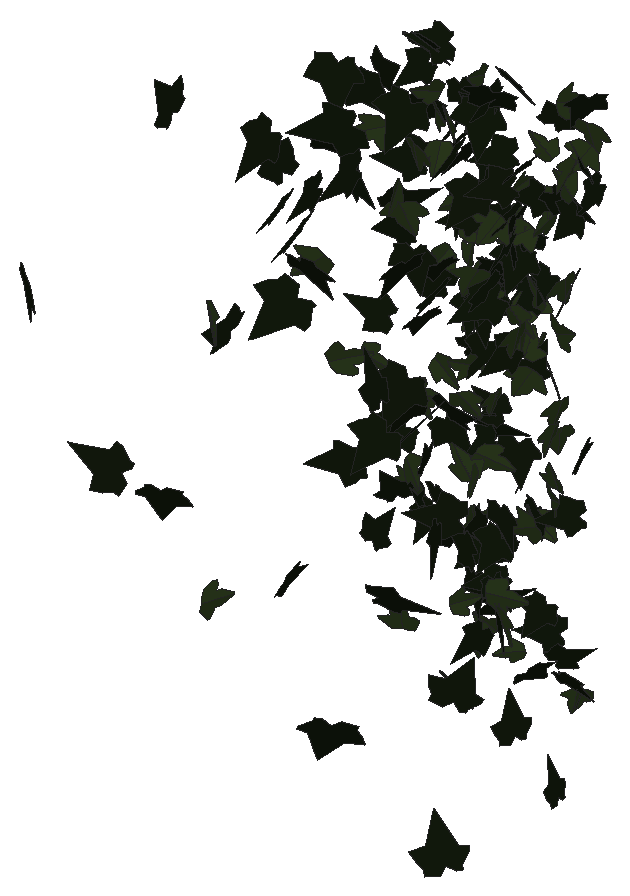
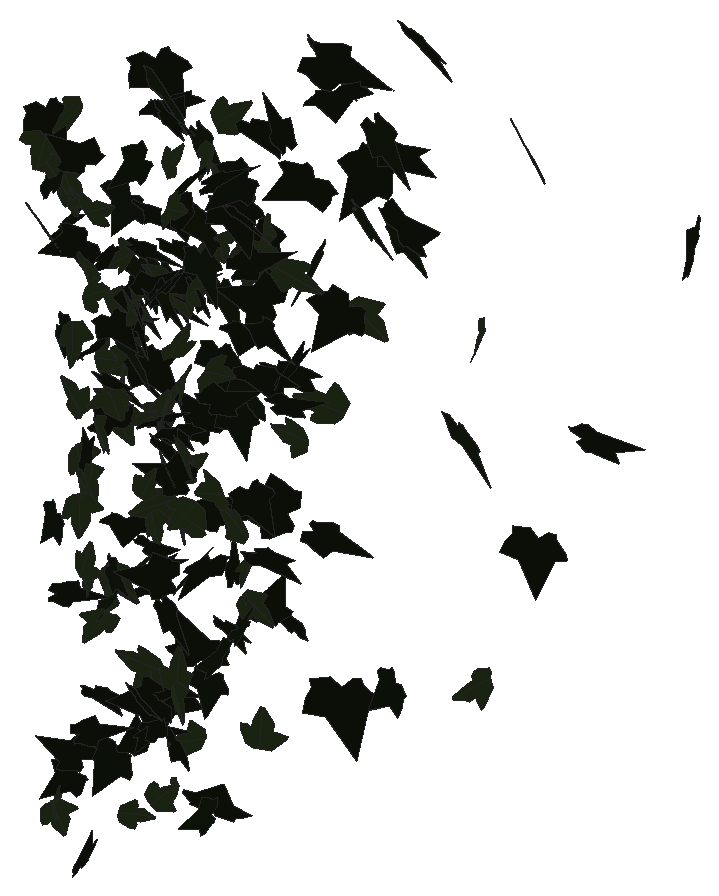
# SketchUp Ruby script. Lengths in millimetres.
U = 1.mm
M = Sketchup.active_model
def pt(a) = Geom::Point3d.new(a.map { |v| v * U })
def face(e, loops, mat)
  f = e.add_face(loops[0].map { |a| pt(a) })
  loops[1..].each { |l| e.add_face(l.map { |a| pt(a) }).erase! }
  f.material = f.back_material = mat if mat
  f
end
# faces: each face lists its corners as indices into pts; further lists are holes
def faces(e, pts, list, mat = nil) = list.each { |f| face(e, (f[0].is_a?(Array) ? f : [f]).map { |l| l.map { |i| pts[i] } }, mat) }
# xy, xz, yz: faces in a plane at the given z, y or x. An outline is a flat list of corners, or four numbers for a rectangle; further outlines are holes
def ring(l) = l.size == 4 ? [[l[0], l[1]], [l[2], l[1]], [l[2], l[3]], [l[0], l[3]]] : l.each_slice(2).to_a
def flat(e, list, mat, &to3) = list.each { |f| face(e, (f[0].is_a?(Array) ? f : [f]).map { |l| ring(l).map { |u, v| to3.(u, v) } }, mat) }
def xy(e, z, list, mat = nil) = flat(e, list, mat) { |x, y| [x, y, z] }
def xz(e, y, list, mat = nil) = flat(e, list, mat) { |x, z| [x, y, z] }
def yz(e, x, list, mat = nil) = flat(e, list, mat) { |y, z| [x, y, z] }
def lines(e, pts, list) = list.each { |a, b| e.add_line(pt(pts[a]), pt(pts[b])) }
# prism: a flat outline (further loops are holes) pulled along v
def prism(e, loops, v, mat = nil)
  f = face(e, loops, mat); d = Geom::Vector3d.new(v.map { |x| x * U })
  f.pushpull(f.normal.samedirection?(d) ? d.length : -d.length)
end
def box(e, o, s, mat = nil) = prism(e, [[o, [o[0] + s[0], o[1], o[2]], [o[0] + s[0], o[1] + s[1], o[2]], [o[0], o[1] + s[1], o[2]]]], [0, 0, s[2]], mat)
def at(x, y, z, deg = 0) = Geom::Transformation.translation(pt([x, y, z])) * Geom::Transformation.rotation(ORIGIN, Z_AXIS, deg.degrees)
def axes(o, x, y, z) = Geom::Transformation.new([*x, 0, *y, 0, *z, 0, *pt(o).to_a, 1])
def part(name) = M.definitions.add(name)
# library, detail: a bought-in or finely detailed component or shape, given as its bounding box
def library(name, o, s) = part(name).tap { |d| box(d.entities, o, s) }
def detail(e, o, s) = box(e.add_group.entities, o, s)
def put(e, d, t, mat = nil) = e.add_instance(d, t).tap { |i| i.material = mat if mat }
def group(e, t, mat = nil) = e.add_group.tap { |g| g.transformation = t; g.material = mat if mat }.entities
root = M.entities
M.materials.add("efeu1").color = [18, 25, 13]
M.materials.add("efeu2").color = [43, 57, 29]
c1 = part("ivyleaf_9")
p = [[39.1,54.8,31.7],[34.5,51.8,30.2],[-5.3,25.2,17.3],[-17.9,28.3,20.9],[-21.6,21.7,17],[-20.2,4.3,5.3],
  [-22.9,-0.3,2.5],[-17.1,-4,-0.6],[-2,-2.1,-1.2],[-0.7,-15.4,-10.1],[16.6,-22.3,-16.7],[21.1,-15.1,-12.5],
  [32.7,-10.7,-11],[46.1,-1.8,-6.6],[30.8,11.2,3.8]]
faces(c1.entities,p,[[0,1,2,3,4,5,6,7,8,9,10,11,12,13,14]],"efeu1")
c2 = part("ivyleaf_10")
p = [[0,12.8,-0.8],[-1.5,51.3,-10.9],[-4.9,51,-11.6],[-13.6,26.5,-7.3],[-13.2,15.9,-4.6],[-21.1,19.3,-7.2],
  [-29.5,16.3,-8.3],[-29.2,8.3,-6.2],[-19.7,-9.8,0.5],[-7.6,-13,4],[1,-12.2,5.8],[-0.4,51.1,-11.1],
  [-1.5,51.1,-10.9],[1,-12.4,5.9],[16.9,-12.4,3.5],[35.1,9.1,-5.1],[35,12.9,-6.1],[20.5,16.4,-4.9],
  [15.8,15,-3.8],[15.3,27.6,-7.1],[12.8,31.3,-7.8]]
faces(c2.entities,p,[[0,1,2,3,4,5,6,7,8,9,10],[11,12,0,13,14,15,16,17,18,19,20]],"efeu2")
put(root,c1,axes([55.6,82.1,1285.6],[0.45869,-0.23293,-1.38227],[1.53626,-0.57264,0.43901],[-0.75134,-1.31306,0.05375]))
put(root,c1,axes([225.6,151.3,899.1],[-1.14115,-0.48465,-0.89648],[-0.97651,-0.4038,1.05345],[-0.76956,1.23107,-0.00739]))
put(root,c1,axes([576.3,245.3,1354.5],[-1.46005,-0.85692,0.36484],[-0.37109,-0.20185,-1.47187],[1.07395,-1.23475,-0.01259]))
put(root,c1,axes([463.1,305.7,1644.5],[-1.71291,0.10789,-0.47473],[0.57263,-0.0846,-1.40741],[-0.15763,-1.47969,0.04586]))
put(root,c1,axes([205.4,303.4,780.9],[1.00786,0.77267,-0.61847],[-0.55474,-0.41924,-1.13113],[-1.07246,0.94298,0.00388]))
put(root,c1,axes([527.4,323.5,1454.6],[-1.0107,1.1156,-0.43445],[0.31599,-0.3488,-1.38956],[-1.426,-0.86799,0.00001]))
put(root,c1,axes([528.1,326.9,1379.9],[1.66772,0.20054,-0.333],[-0.40215,-0.04725,-1.38161],[-0.25136,1.40616,0.00107]))
put(root,c1,axes([582.2,346.2,385.4],[0.82118,1.01451,-0.90267],[-0.64285,-0.73341,-1.21719],[-1.5269,0.85439,0.027]))
put(root,c2,axes([275.1,366.2,1172.6],[-0.51795,1.04749,-0.55022],[0.2633,-0.5062,-1.13022],[-1.41929,-0.47618,-0.00888]))
put(root,c1,axes([620,369,1593.3],[-1.46779,0.67443,-0.22377],[0.23179,-0.11868,-1.37921],[-0.83535,-1.21797,0.01049]))
put(root,c1,axes([686.9,367.3,692.6],[1.08384,-0.27376,1.03511],[1.27629,-0.06449,-0.91492],[0.27817,1.36255,0.16467]))
put(root,c1,axes([174.5,373.7,1565.1],[-0.42554,0.80332,1.20672],[-0.55224,1.11874,-0.8756],[-1.68015,-0.57118,-0.01783]))
put(root,c2,axes([257,379.8,530.6],[-0.05912,-0.19143,-1.2224],[0.57322,1.12885,-0.19541],[1.39643,-0.47149,0.02846]))
put(root,c1,axes([646.6,428.1,1007.3],[-1.48699,-0.57457,-0.02828],[0.02999,0.01418,-1.34748],[0.70119,-1.21909,-0.00234]))
put(root,c1,axes([547.2,445.3,1630.5],[-0.34453,-0.17863,-1.47318],[-1.08704,-1.17881,0.31374],[-1.44778,0.92759,0.11501]))
put(root,c1,axes([792.8,429.2,128.3],[-1.64579,-0.13251,0.15894],[0.19426,0.00487,1.35546],[-0.16125,1.35833,0.01065]))
put(root,c1,axes([366.3,469.9,1386.5],[-0.90124,0.86965,-0.39727],[0.28644,-0.32165,-1.14071],[-1.13071,-0.77464,0.02766]))
put(root,c1,axes([585.6,487.8,1039.8],[-0.40845,-0.99324,0.75452],[0.28417,0.7177,1.04812],[-1.49496,0.40779,-0.00691]))
put(root,c1,axes([229.2,480.3,1060.4],[-0.89362,1.14725,0.43552],[-0.30714,0.35593,-1.361],[-1.46527,-0.77428,0.01967]))
put(root,c1,axes([766.5,488.1,445.8],[-1.05162,-0.07692,0.96033],[1.16947,-0.19731,0.8446],[0.11751,1.27527,0.18861]))
put(root,c1,axes([412.2,514.1,1416.8],[-1.25714,0.56506,-0.40164],[0.406,-0.22803,-1.17459],[-0.74195,-1.08219,0.03779]))
put(root,c1,axes([652.6,489.2,978.4],[-0.30811,1.18465,-0.34746],[-0.08994,0.33955,1.21127],[1.50347,0.26308,0.00126]))
put(root,c1,axes([694.8,524.5,773.9],[-0.81085,0.21669,-1.02259],[1.20492,-0.26673,-0.69844],[-0.4177,-1.19008,-0.02966]))
put(root,c1,axes([610.8,539.4,1061],[-1.48604,-0.67855,-0.32666],[0.34772,0.1596,-1.39432],[0.85043,-1.25097,-0.0007]))
put(root,c1,axes([347.3,505,549.5],[-0.36462,0.48619,-0.98361],[-0.67259,0.81487,0.57029],[1.15735,0.62673,0.02154]))
put(root,c1,axes([613.8,529.9,1317.5],[-0.37333,1.14013,-0.69859],[0.18967,-0.68145,-1.18026],[-1.62024,-0.34248,0.0228]))
put(root,c2,axes([397.8,538.7,1250],[-0.85455,-0.45354,0.88487],[-0.8633,-0.53302,-0.83335],[0.85222,-0.99474,0.0431]))
put(root,c1,axes([318.7,524.2,1423.2],[-0.09591,0.19519,1.39451],[-1.21961,0.97588,-0.19295],[-1.20982,-0.99925,0.08396]))
put(root,c2,axes([446.1,537.5,1047.3],[-0.38963,-0.3588,1.10004],[0.87719,0.83256,0.4803],[-1.106,0.78672,-0.00659]))
put(root,c1,axes([420.8,568,1666.1],[-0.57355,-1.23514,-0.35463],[0.11207,0.34435,-1.32111],[1.56374,-0.4777,-0.03539]))
put(root,c1,axes([458.1,567,822.9],[-0.24261,-0.25527,-1.12314],[-0.9252,-0.82881,0.32265],[-1.05759,0.78362,-0.02461]))
put(root,c1,axes([699.1,577.4,775.7],[-0.74553,-0.13299,1.02767],[-1.23175,-0.19223,-0.62524],[0.28466,-1.18008,-0.01397]))
put(root,c1,axes([484,599,649],[-0.6613,0.57536,0.71293],[0.6009,-0.51545,0.79047],[0.94242,0.73239,-0.00375]))
put(root,c1,axes([638.6,591.8,1232.9],[-0.60337,1.21146,0.07928],[-0.03851,0.07275,-1.30852],[-1.48064,-0.49556,0.00172]))
put(root,c1,axes([648.7,616,974],[0.15352,-0.46219,1.0981],[1.07593,-0.70629,-0.39834],[0.97728,0.85019,0.26604]))
put(root,c2,axes([452.4,621.3,1027],[-0.13538,0.05172,-1.06693],[1.19144,-0.42966,-0.1224],[-0.52796,-0.98287,-0.00263]))
put(root,c1,axes([541.4,634.5,1591.7],[-1.45326,-0.64338,-0.29041],[0.3319,0.10722,-1.35341],[0.79465,-1.22139,0.03416]))
put(root,c2,axes([512,637.7,1400.4],[-0.16625,0.60985,-0.88681],[-0.0257,-0.89523,-0.6124],[-1.3128,-0.0597,0.12429]))
put(root,c1,axes([690.4,633.3,673.7],[0.02582,-1.10176,0.25788],[0.00471,0.25799,1.10193],[-1.38047,-0.01973,0.00858]))
put(root,c1,axes([658.6,626.8,1531.2],[-0.90319,0.84807,-0.33833],[0.27204,-0.25445,-1.12574],[-1.08021,-0.77317,-0.00062]))
put(root,c1,axes([799.1,630.4,321.5],[-0.63448,-0.81045,0.65983],[0.63538,0.43799,0.94846],[-1.1054,0.71694,0.16645]))
put(root,c2,axes([523.6,639,1360.8],[-1.3266,-0.54908,-0.30435],[0.34779,0.11046,-1.2178],[0.68238,-1.12375,0.029]))
put(root,c2,axes([510.8,649.8,450.9],[-1.22373,-0.38729,-0.06213],[-0.07073,-0.02233,1.07523],[-0.47328,1.00473,-0.00005]))
put(root,c1,axes([730.3,634.6,1254.8],[-0.74057,1.1525,0.22615],[-0.19479,0.17124,-1.30117],[-1.41956,-0.62474,0.06056]))
put(root,c1,axes([397.4,637.8,1395.4],[1.01337,-0.60092,-0.79642],[-0.75489,0.50265,-1.0246],[0.95482,1.03517,0.0352]))
put(root,c1,axes([467.3,656.4,1100.5],[-0.79559,-0.58876,-0.57812],[-0.51954,-0.391,0.87857],[-0.86225,0.77884,0.00405]))
put(root,c2,axes([684.7,652.4,829.5],[0.7233,-0.92555,-0.33551],[-0.18829,0.29943,-1.09874],[1.18622,0.61188,0.03017]))
put(root,c1,axes([721.6,667.1,1222.8],[-1.54651,-0.15024,0.27481],[-0.32026,-0.11522,-1.27389],[0.2084,-1.29195,0.08166]))
put(root,c1,axes([678.8,678,480.3],[-0.04303,-0.00885,-1.11829],[0.50108,-1.04076,-0.00472],[-1.26901,-0.41066,0.03605]))
put(root,c2,axes([569.4,678.5,1611.5],[-0.36522,-0.21025,-0.99804],[-0.68633,-0.83358,0.34434],[-1.03794,0.62518,0.12349]))
put(root,c1,axes([521.9,664.3,918.5],[-0.14281,0.80796,-0.71281],[0.07085,-0.71123,-0.81571],[-1.31258,-0.1263,0.03353]))
put(root,c1,axes([442.6,672.1,1611.1],[-0.10981,0.12812,1.13543],[0.66648,-0.99552,0.15564],[1.22437,0.5534,0.01711]))
put(root,c2,axes([675.8,666.7,1259.5],[-0.94431,-0.71989,0.40358],[-0.34974,-0.28432,-1.05698],[0.94417,-0.82532,0.01211]))
put(root,c2,axes([541,657.4,1487],[-1.16669,0.42967,0.2539],[-0.27851,0.11141,-1.04836],[-0.54145,-0.98314,-0.00783]))
put(root,c1,axes([478.5,674.9,709.2],[0.695,0.20223,0.80165],[-0.91902,-0.27424,0.60449],[0.41567,-0.94444,-0.00387]))
put(root,c2,axes([521.7,660.4,794.3],[-0.21545,1.04772,0.235],[-0.0596,0.23007,-1.06245],[-1.30862,-0.18298,0.0097]))
put(root,c1,axes([680.8,682.4,1607.9],[-0.62094,-1.17452,-0.21721],[0.07236,0.21096,-1.27973],[1.45542,-0.51159,-0.02905]))
put(root,c1,axes([716,690.2,687.8],[-0.59263,-0.91416,0.37838],[-0.2331,-0.32691,-1.0351],[1.18431,-0.52179,-0.0144]))
put(root,c1,axes([716.4,666.8,1664.4],[0.33603,0.85581,-0.93751],[-0.85727,-0.69613,-0.84192],[-1.28972,0.6857,0.31536]))
put(root,c2,axes([653.3,672.3,818.7],[1.09321,0.17668,0.6425],[-0.76827,-0.12747,0.91332],[0.26578,-1.09521,-0.00266]))
put(root,c1,axes([511.4,685,1240.2],[-0.68263,-0.66645,-0.66208],[0.54392,0.48992,-0.86994],[1.0088,-0.71512,0.02103]))
put(root,c2,axes([721.4,685.7,530.5],[-1.01545,0.7442,-0.39698],[0.3508,-0.27396,-1.11646],[-0.96738,-0.88053,0.01185]))
put(root,c1,axes([700,673.9,1634],[-0.65096,1.12789,0.44328],[-0.33668,0.35853,-1.24444],[-1.43964,-0.59384,0.09059]))
put(root,c1,axes([377.4,682.3,1568.3],[-0.16498,-0.26499,-1.28924],[1.04585,0.9657,-0.28841],[1.21845,-0.86478,0.07299]))
put(root,c1,axes([470.2,704.5,837.2],[-1.37614,-0.42561,0.12182],[-0.13861,-0.04398,-1.20561],[0.522,-1.13369,0.00104]))
put(root,c1,axes([707.5,704.2,740.8],[0.36569,-1.04193,0.1721],[0.07933,-0.16035,-1.08404],[1.28594,0.30619,0.01793]))
put(root,c2,axes([500.7,693.9,734.6],[-0.60791,-0.14247,0.83957],[-0.99187,-0.20983,-0.51813],[0.30911,-0.95349,-0.01142]))
put(root,c1,axes([523.2,703.6,777.6],[0.0895,0.56182,0.80762],[-0.29982,-0.77373,0.56056],[1.16221,-0.24286,0.08241]))
put(root,c2,axes([678.1,688.7,857.2],[-0.62081,-0.25564,-0.97306],[1.1138,0.34087,-0.56698],[0.51576,-1.04384,0.05315]))
put(root,c2,axes([748.9,700.5,1144],[0.00177,-1.23722,-0.02442],[0.02659,0.02444,-1.23703],[1.50947,0.00102,0.02182]))
put(root,c1,axes([538.2,706,682.2],[-1.10329,-0.11689,-0.34199],[0.4136,0.04499,-0.91186],[0.1528,-0.96579,-0.00109]))
put(root,c1,axes([693.1,712.4,519.5],[-0.19925,0.06873,-1.20253],[1.41227,-0.32635,-0.17587],[-0.40603,-1.16887,-0.02161]))
put(root,c1,axes([682.2,694.3,1590.6],[-0.8831,-0.02588,-0.87365],[-1.06417,-0.05072,0.72421],[-0.06779,1.13343,0.01246]))
put(root,c2,axes([581.1,699.7,1553],[-0.87658,0.75396,-0.07109],[0.05447,-0.05565,-1.04148],[-0.92231,-0.71987,0.00605]))
put(root,c1,axes([736,708.4,1097.9],[-1.43583,0.31113,-0.06093],[0.07018,-0.0208,-1.21733],[-0.38036,-1.1783,0.0054]))
put(root,c1,axes([470.5,707.9,1273.7],[-0.04849,-0.04223,-1.10854],[-1.27469,-0.37134,0.05161],[-0.45482,1.04525,-0.02645]))
put(root,c2,axes([687.7,710.9,550.8],[0.08289,-0.03429,-1.21752],[1.46044,-0.22315,0.07308],[-0.27422,-1.19882,0.02122]))
put(root,c1,axes([515,706.8,1092.7],[-0.02971,1.0361,-0.24756],[0.00953,-0.24744,-1.03639],[-1.29959,-0.0255,-0.00194]))
put(root,c1,axes([451.8,699.6,1314.5],[0.3067,0.03542,1.19047],[1.34231,0.45893,-0.246],[-0.55631,1.12686,0.06277]))
put(root,c1,axes([561.5,719.6,322.9],[0.95523,-0.52366,0.08494],[0.09627,-0.03478,-0.94183],[0.64002,0.7868,0.0149]))
put(root,c1,axes([486.9,719,713.2],[1.05197,-0.73938,-0.36016],[-0.33001,0.23783,-1.13586],[0.94754,0.9037,0.00426]))
put(root,c2,axes([528.2,732.7,1526.7],[-0.29202,0.03101,0.97762],[1.04673,-0.47662,0.22519],[0.57299,0.88649,0.08688]))
put(root,c1,axes([658.5,718.4,680.8],[0.05856,0.03236,-1.17542],[-1.43093,-0.08233,-0.05016],[-0.10201,1.17352,0.02889]))
put(root,c1,axes([618.1,740.4,1383.9],[-1.44381,-0.33009,-0.14086],[0.17366,0.01385,-1.22838],[0.40193,-1.19173,0.02474]))
put(root,c2,axes([483.1,738.9,894.9],[0.54574,-0.25946,-1.05188],[1.08291,-0.56473,0.51678],[-0.75785,-0.99379,-0.01904]))
put(root,c1,axes([473.1,750.8,1396.7],[-0.4812,-0.21627,1.14235],[-1.2046,-0.57459,-0.4497],[0.7489,-1.06319,0.01067]))
put(root,c2,axes([760,730.8,712.3],[-0.6767,-0.00306,0.99705],[-1.20749,-0.13623,-0.55103],[0.14704,-1.13279,0.06358]))
put(root,c1,axes([695.8,740.5,1423.4],[-1.1754,0.00137,0.49421],[-0.6029,0.00887,-0.96341],[-0.00643,-1.08276,-0.00727]))
put(root,c1,axes([603.8,750.9,1318.7],[-0.52669,-0.27867,0.83565],[-0.77468,-0.54656,-0.51031],[0.74486,-0.76549,0.06015]))
put(root,c1,axes([539.9,723.1,1204.8],[0.07795,1.04021,-0.14729],[-0.01814,-0.14665,-1.04216],[-1.28159,0.06535,0.0058]))
put(root,c1,axes([817.7,737.4,148],[-0.16756,-0.85431,0.62675],[0.32086,0.58473,0.85467],[-1.25221,0.26415,0.13513]))
put(root,c1,axes([269.3,724.7,1383.2],[1.19987,0.74184,0.08712],[0.08103,0.05662,-1.2319],[-0.90766,0.98573,0.00519]))
put(root,c2,axes([744.1,739.7,1030.8],[1.25828,0.31187,-0.47094],[-0.65661,0.24508,-1.0164],[-0.20912,1.10701,0.35769]))
put(root,c1,axes([592.5,761.1,1467.2],[-0.61973,0.10068,-0.93521],[0.5813,-0.88887,-0.3545],[-0.98943,-0.58529,0.3775]))
put(root,c2,axes([711.6,764.4,1090.2],[-0.05977,0.07828,1.13161],[0.93231,-0.83476,0.09083],[1.02267,0.76558,-0.01667]))
put(root,c2,axes([654.1,753.4,1326.2],[1.36522,-0.15908,-0.48461],[-0.58475,0.07159,-1.13028],[0.21279,1.21736,0.00314]))
put(root,c2,axes([553.6,770.3,1330.6],[-0.06471,0.11343,1.00782],[0.15506,-1.00049,0.1193],[1.22755,0.13236,0.03806]))
put(root,c2,axes([584,767.6,984.2],[-0.32929,-0.27088,-0.86435],[-0.64917,-0.68247,0.38004],[-0.8943,0.59514,0.0424]))
put(root,c2,axes([370.7,757.5,1428.6],[0.66883,0.08801,-1.01522],[-1.23267,-0.10295,-0.55453],[-0.16165,1.14919,0.02808]))
put(root,c2,axes([516,757.3,1436.3],[0.64298,0.85612,-0.31596],[-0.19857,-0.27083,-1.00533],[-1.09548,0.55158,-0.00321]))
put(root,c2,axes([700.7,755.9,1144.5],[-0.87812,0.24817,-0.71613],[0.81188,-0.26573,-0.76094],[-0.44254,-0.97995,0.02498]))
put(root,c1,axes([657.4,734,509.4],[0.10935,0.84283,-0.82162],[-0.00042,0.82402,0.84525],[1.43599,-0.06394,0.06281]))
put(root,c2,axes([511.3,760.5,964.5],[0.57816,-0.01093,0.96241],[1.17418,-0.00328,-0.47396],[0.00948,1.07276,0.00836]))
put(root,c1,axes([515.8,768.4,1133.9],[-0.18688,0.01192,1.03275],[-1.25515,-0.09368,-0.15152],[0.11093,-1.03984,0.02549]))
put(root,c1,axes([552.8,767.4,1334.9],[-0.75522,0.01098,-0.81012],[0.98715,-0.0437,-0.61887],[-0.05049,-1.01862,0.01782]))
put(root,c2,axes([516.6,776.5,1198.8],[0.32998,0.54148,-0.94122],[-0.49678,-0.84862,-0.60522],[-1.22808,0.48877,-0.00809]))
put(root,c1,axes([698.1,768,851.6],[-0.73463,-0.74922,-0.55206],[0.45556,0.40778,-0.96071],[1.03998,-0.70786,0.03088]))
put(root,c2,axes([568.9,744.9,473.6],[-0.02373,-0.10977,0.97653],[0.1849,0.96469,0.11146],[-1.18452,0.15279,-0.00217]))
put(root,c1,axes([740.8,744.1,384.9],[0.56168,0.96467,0.33598],[0.14517,0.31537,-1.06856],[-1.23775,0.47474,0.02714]))
put(root,c1,axes([534,751.7,604.6],[0.29282,0.89785,0.01121],[0.00335,0.01087,-0.92938],[-1.09546,0.24003,0.00015]))
put(root,c2,axes([570,759.8,914],[-1.0264,-0.15711,-0.51685],[0.61864,0.10011,-0.85584],[0.22722,-0.9823,-0.00456]))
put(root,c1,axes([476.5,761.8,1520.8],[0.71522,0.58152,-0.87248],[-0.78362,-0.59091,-0.82544],[-1.01108,0.86934,0.02256]))
put(root,c2,axes([738.2,766.1,687.3],[-0.91612,0.65629,-0.00469],[-0.01716,-0.00897,0.99717],[0.80051,0.75088,0.01601]))
put(root,c2,axes([775.6,775.6,909],[0.14892,-1.07652,0.27805],[0.11139,-0.26907,-1.08184],[1.35188,0.14076,0.05851]))
put(root,c2,axes([722,765.2,1065.6],[1.22507,-0.13155,-0.12814],[0.15845,0.00515,1.0125],[-0.15839,-1.01228,0.0218]))
put(root,c1,axes([752,780.5,516.3],[-1.10462,-0.38283,-0.11285],[0.12635,0.04485,-0.98303],[0.47024,-0.91133,-0.00097]))
put(root,c1,axes([731,762,1014.8],[-0.57627,-0.31422,0.86097],[0.95259,0.36923,0.56313],[-0.58551,0.90997,0.0688]))
put(root,c1,axes([679.3,759.5,1338.7],[-0.5057,1.0853,0.27622],[-0.17663,0.24013,-1.16076],[-1.35481,-0.4364,0.04823]))
put(root,c1,axes([488.3,783.4,672.3],[0.76587,-0.88077,0.14988],[0.10842,-0.12071,-1.08159],[1.08458,0.63401,0.00229]))
put(root,c1,axes([704.9,753.2,1452.5],[0.31322,0.98822,0.60672],[0.07118,0.60962,-1.01763],[-1.41293,0.24978,0.08324]))
put(root,c1,axes([810.7,799.2,1375.9],[-0.31117,-0.76369,0.73671],[-0.27957,-0.70017,-0.80515],[1.26401,-0.34287,0.00328]))
put(root,c1,axes([668.4,784.7,1286.6],[-1.04577,0.52427,-0.63273],[0.63485,-0.36129,-1.00433],[-0.77585,-1.00229,0.03106]))
put(root,c1,axes([607.9,786,1033.2],[-1.24543,-0.01927,-0.37602],[0.45761,0.04233,-1.02049],[0.0399,-1.08707,-0.03307]))
put(root,c1,axes([592.3,796.1,579.2],[-0.7173,-0.5238,0.40602],[-0.36229,-0.27702,-0.78739],[0.72283,-0.65864,0.00827]))
put(root,c1,axes([635.4,791.8,1311],[0.16012,0.00441,0.93921],[-1.09864,-0.26881,0.1271],[0.32551,-0.90944,-0.03301]))
put(root,c1,axes([518.5,775.1,837.3],[0.24287,-0.73711,-0.86496],[-0.16084,0.85722,-0.76085],[1.37709,0.23012,0.06368]))
put(root,c2,axes([596.4,769.1,381.3],[-0.11648,0.17171,0.87506],[-0.67514,0.67869,-0.19356],[-0.8531,-0.56056,0.0337]))
put(root,c2,axes([779.6,790.6,956.8],[-0.12167,-1.11378,0.12529],[0.00482,-0.12613,-1.11814],[1.36738,-0.09866,0.01509]))
put(root,c1,axes([676.4,802.9,1243.7],[-0.71139,-1.01327,0.05954],[0.02891,-0.08224,-1.16746],[1.23799,-0.58034,0.06148]))
put(root,c1,axes([527.5,766.1,1462.1],[-0.57681,0.84163,-0.58854],[-0.40543,0.48768,0.96436],[1.18553,0.57627,0.04345]))
put(root,c1,axes([538.4,792.7,1564.3],[0.33517,-0.90215,-0.28451],[-0.09518,0.27365,-0.94304],[1.15013,0.28555,0.00487]))
put(root,c1,axes([602.6,809.4,809.6],[-0.48928,-0.5135,0.6804],[-0.4275,-0.58616,-0.64892],[0.94803,-0.52934,0.05854]))
put(root,c2,axes([792.5,809.7,1470.1],[0.01876,-0.78988,0.75027],[0.20034,-0.74009,-0.78253],[1.31389,0.12412,0.1086]))
put(root,c2,axes([809.6,785.1,1432.1],[0.50584,0.06343,1.02926],[-1.22441,0.27973,0.38706],[-0.28909,-1.0738,0.16163]))
put(root,c1,axes([708.6,810.4,698.6],[0.23766,-0.82397,0.50147],[0.15515,-0.48519,-0.84662],[1.1665,0.2324,0.01043]))
put(root,c1,axes([667.2,784.7,1270.6],[0.23802,-0.0134,-1.18093],[-1.42855,0.15371,-0.19519],[0.18768,1.18703,0.01194]))
put(root,c2,axes([575,805.3,985.5],[0.48715,-0.50089,-0.65183],[0.53793,-0.4811,0.6398],[-0.84643,-0.59403,0.03146]))
put(root,c1,axes([757,812,446.1],[-0.53423,-0.1826,0.92619],[-1.04799,-0.34637,-0.47441],[0.47765,-0.96416,-0.00498]))
put(root,c2,axes([569.6,818.6,1585.1],[-0.06648,-0.30842,-0.89808],[-0.16606,-0.88773,0.31313],[-1.14651,0.14646,0.00672]))
put(root,c2,axes([558.6,811.8,615.5],[-0.34286,-0.94674,-0.41689],[-0.07896,-0.41507,0.98622],[-1.25958,0.28373,0.05165]))
put(root,c2,axes([745.8,810.2,728.8],[-0.52038,0.23922,0.82716],[0.89912,-0.37594,0.48876],[0.54325,0.85136,-0.0166]))
put(root,c1,axes([562.1,809.4,501],[-0.69369,-0.00907,-0.92129],[1.12393,0.00792,-0.56866],[0.01403,-1.08259,0.00356]))
put(root,c2,axes([683.4,806.5,1293.9],[0.89229,0.04132,-0.84086],[-1.02214,-0.07346,-0.73235],[-0.10068,1.11201,-0.01714]))
put(root,c1,axes([631.2,800.7,1191.6],[0.08441,0.53824,-1.02259],[-1.05914,-0.65192,-0.40188],[-0.9305,0.79087,0.36467]))
put(root,c1,axes([570.4,813.9,1091.1],[-0.73509,-0.44485,-0.79269],[0.9662,0.20986,-0.71976],[0.54429,-0.97333,0.20711]))
put(root,c2,axes([566.4,819.8,1506.9],[0.07722,0.53285,-0.84283],[-0.27693,-0.81465,-0.53209],[-1.18458,0.22518,0.06945]))
put(root,c1,axes([614.4,819.9,505.2],[-0.65048,-0.26031,0.69488],[-0.76565,-0.29836,-0.59331],[0.48302,-0.82348,-0.00469]))
put(root,c1,axes([662,784.6,1285.9],[0.10877,0.08245,1.19053],[0.50313,1.11817,-0.10832],[-1.36623,0.41834,0.05489]))
put(root,c1,axes([555,819.3,1094.7],[-0.63952,-0.82587,-0.14831],[0.10152,0.12284,-0.97817],[1.01863,-0.53074,0.00438]))
put(root,c1,axes([673.3,797.8,1213.5],[-0.64038,1.0271,0.21942],[-0.14156,0.18708,-1.15332],[-1.27349,-0.53727,0.01787]))
put(root,c1,axes([514.4,801.1,1427],[-0.34834,1.10913,-0.1052],[0.03373,-0.10151,-1.14529],[-1.3588,-0.28685,-0.00146]))
put(root,c1,axes([608.1,808.8,508.1],[0.12406,-0.67946,-0.53104],[-0.06124,0.52915,-0.68665],[1.0503,0.11111,0.02269]))
put(root,c1,axes([702.2,830.4,1365.4],[0.06385,-0.73378,-0.62109],[0.19345,-0.60691,0.73038],[-1.15679,-0.14199,0.08786]))
put(root,c1,axes([777.2,803.8,362.3],[1.17368,0.02659,0.05862],[0.07153,0.0003,-0.9624],[-0.0324,0.96382,-0.00132]))
put(root,c1,axes([793.3,826,704.2],[-0.77531,-0.23943,0.76644],[-0.87927,-0.26087,-0.67908],[0.43192,-0.96085,-0.00662]))
put(root,c2,axes([603.8,815.2,905.1],[0.02003,-0.94734,0.01205],[0.01304,-0.01187,-0.94742],[1.15577,0.01655,0.01048]))
put(root,c1,axes([767.7,804.5,394.4],[0.15742,-0.08419,0.94172],[1.14699,0.11211,-0.1188],[-0.12219,0.94388,0.0981]))
put(root,c2,axes([724.7,800.8,1162.1],[-0.37811,0.35557,-0.99241],[-0.86501,0.69518,0.47051],[0.95176,0.77309,0.03336]))
put(root,c1,axes([549.6,806,994.6],[0.43356,-0.03163,0.93868],[1.14582,0.01745,-0.35499],[-0.00625,1.00355,0.03575]))
put(root,c1,axes([804.8,832.6,1469.4],[-0.24952,-0.30982,1.0056],[0.26207,-1.01514,-0.26907],[1.2567,0.15018,0.25578]))
put(root,c1,axes([732.6,830.6,977.7],[0.04463,-0.25986,0.90874],[0.22682,-0.88967,-0.26189],[1.13057,0.18875,0.01667]))
put(root,c2,axes([761,814.3,881.3],[-0.53378,-0.99419,-0.09924],[0.02186,0.10052,-1.08594],[1.21875,-0.43723,-0.02399]))
put(root,c2,axes([748.6,816.4,762.1],[-1.09935,0.31606,-0.08277],[-0.09678,0.02391,0.95492],[0.38667,0.90459,0.00368]))
put(root,c1,axes([721.1,833.9,1195.6],[-0.3012,-0.83209,0.37404],[-0.08523,-0.36911,-0.86724],[1.10973,-0.25419,0.03491]))
put(root,c2,axes([555.7,817.4,1240.4],[0.21722,1.02887,0.22739],[-0.05939,-0.22234,1.04411],[1.28413,-0.18432,0.00983]))
put(root,c2,axes([546.1,818.1,1066.8],[0.98212,-0.64729,-0.2514],[-0.23925,0.1573,-1.03297],[0.81268,0.82856,-0.00029]))
put(root,c2,axes([712.3,806.3,677.7],[0.51075,0.75372,0.61853],[0.34538,0.55018,-0.86203],[-1.13829,0.50513,0.01598]))
put(root,c1,axes([584.1,836,1339.4],[-0.1511,-0.18483,0.88129],[-0.5862,-0.73878,-0.22247],[0.92909,-0.49619,0.00296]))
put(root,c2,axes([590.2,809.5,1110.3],[-0.47586,-0.289,-0.83354],[0.90844,0.38091,-0.48051],[0.57721,-0.83776,0.06907]))
put(root,c1,axes([684.7,826.9,791.9],[-0.66453,0.44355,-0.68773],[0.65245,-0.4324,-0.70244],[-0.75571,-0.76334,-0.00171]))
put(root,c2,axes([818.3,822.2,1508],[1.25199,-0.09184,-0.47066],[-0.56857,0.07092,-1.02999],[0.13784,1.12678,0.02647]))
put(root,c2,axes([781.3,800.1,1609.1],[-0.06175,0.34907,1.048],[-0.26148,1.02606,-0.35211],[-1.32201,-0.21925,0.02069]))
put(root,c1,axes([576.8,827,1344.1],[-0.87983,0.54407,-0.54667],[0.53629,-0.32502,-0.90338],[-0.77317,-0.84457,-0.00451]))
put(root,c2,axes([587.1,828,389.7],[-0.69516,-0.12119,-0.60933],[-0.71299,-0.17597,0.5815],[-0.25717,0.81547,0.03493]))
put(root,c1,axes([783.9,831,1212.6],[-0.72487,0.49067,-0.79124],[0.73428,-0.51371,-0.77052],[-0.8666,-0.84569,0.00897]))
put(root,c2,axes([634.8,834.7,1297.8],[-0.04684,-0.0636,-0.9919],[0.80911,-0.74099,0.02184],[-0.90318,-0.66051,0.071]))
put(root,c2,axes([768.3,820.4,1205.5],[-0.2222,-1.09237,-0.28856],[0.08081,0.28145,-1.1073],[1.37604,-0.19292,0.01843]))
put(root,c1,axes([425.8,831.4,1557.5],[-1.33338,0.11233,-0.02551],[0.02344,-0.06221,-1.09706],[-0.13856,-1.09146,0.0599]))
put(root,c2,axes([570.2,814.2,1140.4],[-0.05214,0.8381,0.37468],[-0.0571,0.37261,-0.83881],[-1.11855,-0.05809,0.02535]))
put(root,c1,axes([412.2,815.1,1614.4],[1.36743,0.05707,0.01287],[0.0135,0.03564,-1.12175],[-0.07009,1.12035,0.03503]))
put(root,c1,axes([573.8,843.3,1116.1],[-0.60042,-0.97903,0.15984],[0.13135,-0.23009,-1.07783],[1.20308,-0.46349,0.19745]))
put(root,c2,axes([701.3,835.7,1050],[0.59354,-0.86769,0.40606],[0.24042,-0.35504,-0.99477],[1.14376,0.5249,-0.00161]))
put(root,c1,axes([689.8,833.6,1150.6],[-1.36958,0.03762,0.0796],[-0.09807,-0.02268,-1.12295],[-0.04381,-1.12519,0.0253]))
put(root,c2,axes([544.5,807,1185.6],[0.02137,0.40215,-0.91438],[-0.11003,0.91142,0.39912],[1.21369,0.07555,0.05228]))
put(root,c2,axes([666.3,807.9,1379.1],[0.104,-0.0547,0.92635],[-0.29794,0.89614,0.07539],[-1.09221,-0.24966,0.06764]))
put(root,c2,axes([787.3,842.2,313.3],[0.02957,-0.06206,0.92116],[0.675,-0.73671,-0.06419],[0.90171,0.55352,0.01784]))
put(root,c2,axes([743.9,834.9,1077.8],[-0.75615,0.09958,0.90641],[1.08442,-0.1786,0.62742],[0.24825,1.08343,0.02012]))
put(root,c1,axes([675.9,834.6,1267],[0.10722,0.45969,-0.76832],[-0.22949,-0.7453,-0.46744],[-1.06793,0.20631,0.02331]))
put(root,c2,axes([562.6,827.2,1159.4],[-0.00193,1.1336,-0.02411],[0.00583,-0.0241,-1.13359],[-1.38329,-0.00169,-0.00474]))
put(root,c1,axes([621.6,837.8,1423.5],[-1.08349,0.06353,0.49285],[-0.60443,-0.035,-0.88825],[-0.04697,-1.01509,0.06147]))
put(root,c1,axes([457.2,849.5,1604.5],[-0.14853,-0.90105,-0.60518],[-0.1166,-0.59771,0.90915],[-1.31907,0.15429,-0.01222]))
put(root,c2,axes([638.2,842.9,352.2],[-0.11839,-0.06481,0.81421],[-0.52767,-0.69146,-0.10659],[0.8453,-0.44072,0.0475]))
put(root,c1,axes([742.7,824.1,1384.5],[0.01431,0.03628,-1.07188],[0.94138,0.7442,0.03363],[0.90874,-0.77151,-0.01796]))
put(root,c2,axes([824,828.7,1555.5],[-1.37855,0.05466,-0.05608],[0.06876,0.00448,-1.13126],[-0.06633,-1.13134,-0.00719]))
put(root,c1,axes([814.8,833.1,1612.5],[0.15322,0.81604,-0.69572],[-0.08837,-0.69242,-0.82525],[-1.30529,0.14266,-0.0258]))
put(root,c2,axes([564.2,830,1153.2],[0.25662,1.10925,0.00632],[0.00389,0.00583,-1.12901],[-1.3533,0.21036,-0.00205]))
put(root,c2,axes([706.7,853.5,1308.3],[-0.00814,-0.17973,1.03263],[0.33263,-0.9974,-0.17184],[1.23473,0.26751,0.0531]))
put(root,c1,axes([604.3,832.7,861.1],[-0.92819,-0.26147,-0.45926],[-0.51902,-0.17457,0.80415],[-0.38251,0.87137,0.02329]))
put(root,c2,axes([598.1,849.1,977.4],[-0.33657,-0.54853,-0.61969],[-0.33652,-0.55492,0.61399],[-0.95192,0.39012,0.00205]))
put(root,c1,axes([810.4,815.6,842.8],[-0.31969,0.36444,-0.95279],[-0.84707,0.65698,0.44225],[0.91178,0.73814,0.0768]))
put(root,c2,axes([671.8,841.9,1124.5],[0.89925,0.75243,-0.3262],[-0.255,-0.25176,-1.05299],[-0.96748,0.76572,-0.02566]))
put(root,c2,axes([535.4,840.2,613.9],[0.35174,-0.97294,-0.02223],[-0.00241,0.0226,-1.01475],[1.1873,0.28829,0.00453]))
put(root,c1,axes([561.1,860,1366.8],[-0.18738,-0.87286,0.61171],[-0.09769,-0.60683,-0.886],[1.29668,-0.17185,0.02164]))
put(root,c1,axes([626.3,830,569.4],[-0.45191,0.47129,0.68245],[-0.54803,0.51429,-0.59899],[-0.85057,-0.58177,0.02335]))
put(root,c1,axes([738.3,831.1,1539],[-0.2366,-0.11076,1.00396],[1.20809,0.18065,0.21121],[-0.24289,1.00643,0.07258]))
put(root,c2,axes([788.1,846,310.7],[-0.59058,-0.72056,0.30516],[-0.18549,-0.26539,-0.86782],[0.93647,-0.50698,0.02056]))
put(root,c1,axes([559.2,834.5,818.2],[0.82144,-0.03723,0.82201],[1.00039,-0.05809,-0.67429],[0.08359,1.06098,-0.00808]))
put(root,c2,axes([713.6,841.3,1458.2],[0.70973,0.12471,0.73637],[-0.8763,-0.16232,0.59494],[0.24965,-0.9243,-0.00512]))
put(root,c2,axes([555.9,840.9,1153],[-0.68381,0.95467,-0.11474],[0.06298,-0.10275,-1.10702],[-1.17139,-0.56283,0.00746]))
put(root,c1,axes([607.6,839.8,1592],[1.24647,-0.22836,-0.10217],[-0.11383,0.05079,-1.0465],[0.28319,1.02554,0.02908]))
put(root,c1,axes([824,852.6,1419.6],[-1.16201,0.29765,-0.41369],[0.4768,-0.13621,-0.99781],[-0.39906,-1.02945,0.01241]))
put(root,c2,axes([715.9,851,1365.3],[1.02833,-0.38723,0.13799],[0.15406,-0.05566,-0.92758],[0.47726,0.8523,0.00212]))
